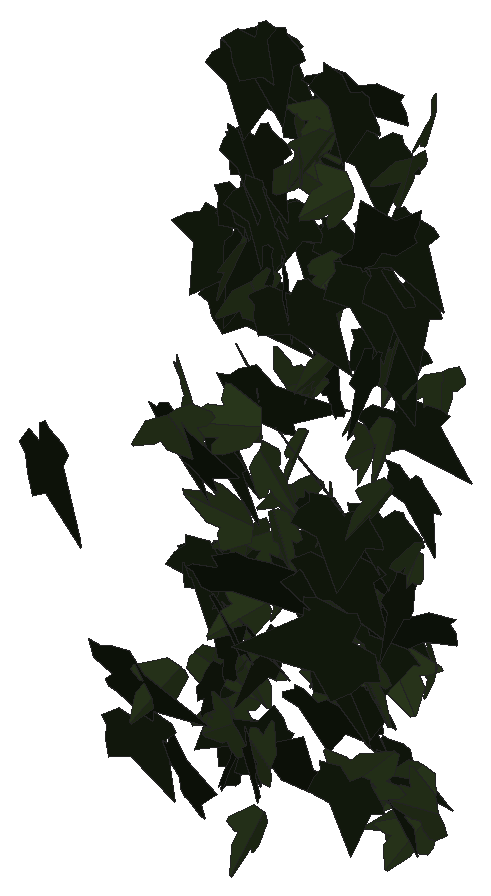
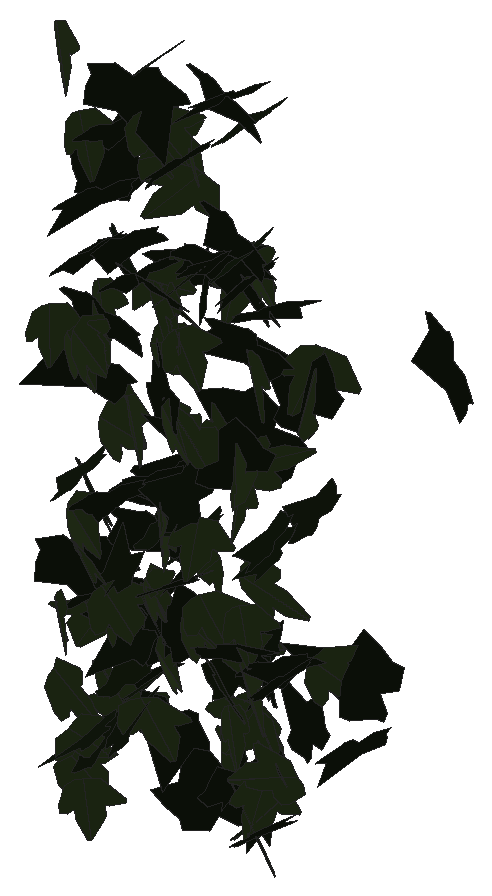
# SketchUp Ruby script. Lengths in inches.
U = 1.inch
M = Sketchup.active_model
def pt(a) = Geom::Point3d.new(a.map { |v| v * U })
def face(e, loops, mat)
  f = e.add_face(loops[0].map { |a| pt(a) })
  loops[1..].each { |l| e.add_face(l.map { |a| pt(a) }).erase! }
  f.material = f.back_material = mat if mat
  f
end
# faces: each face lists its corners as indices into pts; further lists are holes
def faces(e, pts, list, mat = nil) = list.each { |f| face(e, (f[0].is_a?(Array) ? f : [f]).map { |l| l.map { |i| pts[i] } }, mat) }
# xy, xz, yz: faces in a plane at the given z, y or x. An outline is a flat list of corners, or four numbers for a rectangle; further outlines are holes
def ring(l) = l.size == 4 ? [[l[0], l[1]], [l[2], l[1]], [l[2], l[3]], [l[0], l[3]]] : l.each_slice(2).to_a
def flat(e, list, mat, &to3) = list.each { |f| face(e, (f[0].is_a?(Array) ? f : [f]).map { |l| ring(l).map { |u, v| to3.(u, v) } }, mat) }
def xy(e, z, list, mat = nil) = flat(e, list, mat) { |x, y| [x, y, z] }
def xz(e, y, list, mat = nil) = flat(e, list, mat) { |x, z| [x, y, z] }
def yz(e, x, list, mat = nil) = flat(e, list, mat) { |y, z| [x, y, z] }
def lines(e, pts, list) = list.each { |a, b| e.add_line(pt(pts[a]), pt(pts[b])) }
# prism: a flat outline (further loops are holes) pulled along v
def prism(e, loops, v, mat = nil)
  f = face(e, loops, mat); d = Geom::Vector3d.new(v.map { |x| x * U })
  f.pushpull(f.normal.samedirection?(d) ? d.length : -d.length)
end
def box(e, o, s, mat = nil) = prism(e, [[o, [o[0] + s[0], o[1], o[2]], [o[0] + s[0], o[1] + s[1], o[2]], [o[0], o[1] + s[1], o[2]]]], [0, 0, s[2]], mat)
def at(x, y, z, deg = 0) = Geom::Transformation.translation(pt([x, y, z])) * Geom::Transformation.rotation(ORIGIN, Z_AXIS, deg.degrees)
def axes(o, x, y, z) = Geom::Transformation.new([*x, 0, *y, 0, *z, 0, *pt(o).to_a, 1])
def part(name) = M.definitions.add(name)
# library, detail: a bought-in or finely detailed component or shape, given as its bounding box
def library(name, o, s) = part(name).tap { |d| box(d.entities, o, s) }
def detail(e, o, s) = box(e.add_group.entities, o, s)
def put(e, d, t, mat = nil) = e.add_instance(d, t).tap { |i| i.material = mat if mat }
def group(e, t, mat = nil) = e.add_group.tap { |g| g.transformation = t; g.material = mat if mat }.entities
root = M.entities
M.materials.add("1026 AP 7946 SUNNY SIDE UP").color = [254, 231, 186]
M.materials.add("efeu1").color = [18, 25, 13]
M.materials.add("efeu2").color = [43, 57, 29]
c1 = part("ivyleaf_9")
p = [[1.54,2.16,1.25],[1.36,2.04,1.19],[-0.21,0.99,0.68],[-0.71,1.11,0.82],[-0.85,0.86,0.67],[-0.8,0.17,0.21],
  [-0.9,-0.01,0.1],[-0.67,-0.16,-0.02],[-0.08,-0.08,-0.05],[-0.03,-0.6,-0.4],[0.65,-0.88,-0.66],[0.83,-0.6,-0.49],
  [1.29,-0.42,-0.43],[1.8125,-0.07,-0.26],[1.21,0.44,0.15]]
faces(c1.entities,p,[[0,1,2,3,4,5,6,7,8,9,10,11,12,13,14]],"efeu1")
c2 = part("ivyleaf_10")
p = [[0,0.5,-0.03],[-0.0625,2.02,-0.43],[-0.19,2.01,-0.46],[-0.54,1.05,-0.29],[-0.52,0.625,-0.18],[-0.83,0.76,-0.28],
  [-1.16,0.64,-0.33],[-1.15,0.33,-0.24],[-0.77,-0.39,0.02],[-0.3,-0.51,0.16],[0.04,-0.48,0.23],[-0.02,2.01,-0.4375],
  [-0.06,2.01,-0.43],[0.04,-0.49,0.23],[0.67,-0.49,0.14],[1.38,0.36,-0.2],[1.375,0.51,-0.24],[0.81,0.65,-0.19],
  [0.62,0.59,-0.15],[0.6,1.09,-0.28],[0.5,1.23,-0.31]]
faces(c2.entities,p,[[0,1,2,3,4,5,6,7,8,9,10],[11,12,0,13,14,15,16,17,18,19,20]],"efeu2")
put(root,c1,axes([121.61,208.34,285.75],[-0.09102,-0.03713,-0.47993],[0.72895,-0.06226,-0.05462],[-0.09031,-0.46509,0.04284]),"1026 AP 7946 SUNNY SIDE UP")
put(root,c1,axes([124.05,209.3,284.24],[0.61403,0.15623,0.13736],[0.21568,0.01226,-0.43147],[-0.23915,0.41217,-0.03647]),"1026 AP 7946 SUNNY SIDE UP")
put(root,c2,axes([124.125,209.9,279.97],[-0.01613,-0.25056,0.28133],[0.13214,-0.26906,-0.25135],[0.56927,0.05536,0.06631]),"1026 AP 7946 SUNNY SIDE UP")
put(root,c1,axes([125.59,210.1,283.27],[-0.05091,-0.26888,-0.37248],[-0.09121,-0.35545,0.27677],[-0.70066,0.06581,-0.00896]),"1026 AP 7946 SUNNY SIDE UP")
put(root,c2,axes([122.8,209.76,285.93],[-0.33022,-0.28248,-0.17885],[0.18974,0.12426,-0.36128],[0.48418,-0.24135,0.0196]),"1026 AP 7946 SUNNY SIDE UP")
put(root,c1,axes([122.71,210.06,280.16],[0.05579,-0.04879,0.37356],[0.17873,-0.34511,-0.06127],[0.5473,0.11767,-0.01807]),"1026 AP 7946 SUNNY SIDE UP")
put(root,c1,axes([122.64,210.1,285.39],[0.10603,-0.13519,0.41887],[0.32724,-0.35034,-0.15732],[0.59024,0.21852,0.01198]),"1026 AP 7946 SUNNY SIDE UP")
put(root,c1,axes([121.55,210.08,281.34],[0.32519,-0.12393,0.35637],[0.40668,-0.234,-0.24653],[0.41189,0.32888,-0.03794]),"1026 AP 7946 SUNNY SIDE UP")
put(root,c2,axes([122.31,210.27,281.5],[-0.11299,-0.24724,0.28312],[0.00223,-0.28155,-0.26088],[0.58291,-0.04684,0.05588]),"1026 AP 7946 SUNNY SIDE UP")
put(root,c1,axes([121.69,210.31,280.56],[0.08574,-0.31958,-0.16892],[-0.03577,0.1606,-0.33303],[0.56236,0.05894,0.00457]),"1026 AP 7946 SUNNY SIDE UP")
put(root,c1,axes([125.13,210.74,280.59],[-0.08001,-0.32564,0.01922],[-0.0008,-0.02068,-0.33965],[0.51305,-0.05081,0.00247]),"1026 AP 7946 SUNNY SIDE UP")
put(root,c1,axes([125.38,210.9,287.25],[-0.30488,0.04205,-0.31612],[0.42375,-0.15608,-0.19822],[-0.24078,-0.32793,0.05142]),"1026 AP 7946 SUNNY SIDE UP")
put(root,c2,axes([122.25,210.77,285.64],[-0.31836,0.30173,0.0568],[0.06922,-0.03472,0.37372],[0.47682,0.2065,-0.01633]),"1026 AP 7946 SUNNY SIDE UP")
put(root,c1,axes([123.96,211,283.3125],[0.12499,-0.33358,0.08934],[0.02003,-0.08804,-0.3537],[0.54235,0.08013,-0.00753]),"1026 AP 7946 SUNNY SIDE UP")
put(root,c2,axes([123.43,210.98,284.96],[0.17881,-0.04143,0.34507],[0.48767,-0.12721,-0.12534],[0.21025,0.3303,-0.00274]),"1026 AP 7946 SUNNY SIDE UP")
put(root,c2,axes([123.31,210.86,287.73],[-0.17253,-0.34111,-0.16611],[0.11104,0.14434,-0.36766],[0.58147,-0.12878,0.02092]),"1026 AP 7946 SUNNY SIDE UP")
put(root,c2,axes([122.92,210.86,280.68],[-0.27788,0.1153,0.25612],[-0.38362,0.06688,-0.21077],[-0.19422,-0.29706,0.04987]),"1026 AP 7946 SUNNY SIDE UP")
put(root,c1,axes([123.12,211.16,279.85],[-0.11226,0.0883,0.32367],[-0.09416,-0.31921,0.07666],[0.50368,-0.03999,0.08647]),"1026 AP 7946 SUNNY SIDE UP")
put(root,c2,axes([122.85,211.11,288.04],[0.14731,-0.33648,0.0969],[0.03265,-0.09383,-0.36034],[0.54921,0.09583,-0.00457]),"1026 AP 7946 SUNNY SIDE UP")
put(root,c1,axes([124.27,211.32,282.44],[-0.11251,-0.16508,0.3382],[-0.17941,-0.30894,-0.18694],[0.55061,-0.1344,0.00819]),"1026 AP 7946 SUNNY SIDE UP")
put(root,c1,axes([122.62,211.26,281.99],[-0.00972,-0.15483,0.29514],[0.08362,-0.28406,-0.15815],[0.50641,0.04393,0.03178]),"1026 AP 7946 SUNNY SIDE UP")
put(root,c1,axes([123.89,211.04,287.7],[-0.08042,-0.21821,-0.29571],[0.23162,0.25063,-0.22283],[0.51579,-0.14657,0.05396]),"1026 AP 7946 SUNNY SIDE UP")
put(root,c1,axes([125.73,211.19,283.64],[-0.34251,0.07972,-0.26507],[0.36347,-0.11571,-0.23879],[-0.2188,-0.31702,0.01828]),"1026 AP 7946 SUNNY SIDE UP")
put(root,c1,axes([122.57,211.18,281.49],[-0.07866,0.1721,0.28129],[0.04264,-0.2721,0.18086],[0.5044,0.04984,0.02858]),"1026 AP 7946 SUNNY SIDE UP")
put(root,c2,axes([125.02,211.21,282.23],[-0.35779,0.22008,-0.21852],[0.20305,-0.17217,-0.32583],[-0.43712,-0.26011,0.02751]),"1026 AP 7946 SUNNY SIDE UP")
put(root,c1,axes([121.57,211.33,284.63],[0.18205,-0.29227,0.14544],[0.0786,-0.13383,-0.32463],[0.50543,0.12608,-0.00191]),"1026 AP 7946 SUNNY SIDE UP")
put(root,c1,axes([123.53,211.4,287.3],[-0.01971,0.02165,0.38698],[-0.06805,-0.37331,0.0185],[0.58752,-0.04251,0.01513]),"1026 AP 7946 SUNNY SIDE UP")
put(root,c2,axes([125.13,211.41,284.87],[0.04592,-0.23723,0.27759],[0.04198,-0.26951,-0.24778],[0.56453,0.03934,-0.00415]),"1026 AP 7946 SUNNY SIDE UP")
put(root,c2,axes([124.37,211.47,289.33],[-0.1084,-0.02226,0.36682],[0.06144,-0.36107,-0.01757],[0.5578,0.03544,0.07322]),"1026 AP 7946 SUNNY SIDE UP")
put(root,c2,axes([122.66,211.45,285.09],[-0.0318,0.11349,0.38625],[-0.16041,-0.36334,0.10569],[0.5937,-0.09209,0.04924]),"1026 AP 7946 SUNNY SIDE UP")
put(root,c2,axes([122.85,211.48,282.24],[-0.11298,-0.10099,0.33685],[-0.03896,-0.33227,-0.11308],[0.53756,-0.04531,0.0626]),"1026 AP 7946 SUNNY SIDE UP")
put(root,c1,axes([122.92,211.375,287.95],[-0.46652,0.03473,-0.23776],[0.35274,-0.0617,-0.30676],[-0.10236,-0.37091,0.02652]),"1026 AP 7946 SUNNY SIDE UP")
put(root,c1,axes([124.46,211.4375,284.27],[-0.19498,-0.32406,-0.01834],[0.0232,0.01144,-0.35725],[0.50965,-0.1245,0.00924]),"1026 AP 7946 SUNNY SIDE UP")
put(root,c2,axes([124.9,211.26,280.34],[-0.46007,-0.10063,0.17273],[0.23059,0.08822,0.31762],[-0.20455,0.32578,-0.03043]),"1026 AP 7946 SUNNY SIDE UP")
put(root,c2,axes([123.67,211.45,285.16],[0.26307,-0.30067,0.14705],[0.08531,-0.13491,-0.35484],[0.51752,0.17508,-0.01626]),"1026 AP 7946 SUNNY SIDE UP")
put(root,c2,axes([123.38,211.11,280.17],[0.07023,0.03151,0.37937],[-0.49688,0.19531,0.02342],[-0.30089,-0.31517,0.04988]),"1026 AP 7946 SUNNY SIDE UP")
put(root,c2,axes([124.07,211.59,286.59],[0.04814,-0.08331,0.37593],[0.13547,-0.35522,-0.09295],[0.57349,0.0909,-0.0096]),"1026 AP 7946 SUNNY SIDE UP")
put(root,c2,axes([125.22,211.42,285.89],[0.33467,-0.24235,0.11131],[0.10141,-0.08893,-0.33266],[0.40563,0.22219,-0.00867]),"1026 AP 7946 SUNNY SIDE UP")
put(root,c2,axes([126.18,211.2,280.34],[-0.19311,0.05531,0.37011],[-0.55424,0.07316,-0.13543],[-0.13763,-0.37225,0.02607]),"1026 AP 7946 SUNNY SIDE UP")
put(root,c1,axes([125.12,211.46,288.7],[0.25256,0.17382,0.33773],[-0.39064,-0.21352,0.24151],[0.43153,-0.29502,0.02096]),"1026 AP 7946 SUNNY SIDE UP")
put(root,c2,axes([124.34,211.43,282.6],[0.22254,-0.3072,0.06021],[0.01862,-0.06076,-0.34849],[0.49188,0.14129,-0.01405]),"1026 AP 7946 SUNNY SIDE UP")
put(root,c1,axes([122.79,211.54,281.7],[0.45271,-0.21313,-0.08655],[0.13142,-0.02584,0.36773],[-0.33465,-0.29847,0.02733]),"1026 AP 7946 SUNNY SIDE UP")
put(root,c1,axes([124.32,211.38,283.48],[-0.12408,-0.16562,-0.31602],[0.40093,0.18571,-0.1703],[0.3719,-0.25547,0.07816]),"1026 AP 7946 SUNNY SIDE UP")
put(root,c1,axes([122.6,211.67,290.54],[-0.07719,-0.32886,0.16903],[0.02267,-0.169,-0.34162],[0.57877,-0.03724,0.03593]),"1026 AP 7946 SUNNY SIDE UP")
put(root,c1,axes([124.39,211.66,290.82],[-0.05839,-0.33295,0.15199],[-0.01346,-0.14936,-0.34592],[0.57368,-0.03739,0.00735]),"1026 AP 7946 SUNNY SIDE UP")
put(root,c1,axes([122.24,211.72,287.8],[-0.30862,-0.27455,0.11321],[-0.03626,-0.11913,-0.34485],[0.46451,-0.19171,0.0483]),"1026 AP 7946 SUNNY SIDE UP")
put(root,c2,axes([123.875,211.66,289.89],[-0.01015,-0.2992,0.21085],[0.00111,-0.20641,-0.30949],[0.57152,-0.00492,0.00435]),"1026 AP 7946 SUNNY SIDE UP")
put(root,c1,axes([123.11,211.59,281.64],[-0.40042,0.10925,-0.19393],[0.25342,-0.10149,-0.28494],[-0.23127,-0.30037,0.02356]),"1026 AP 7946 SUNNY SIDE UP")
put(root,c2,axes([123.45,211.73,289.86],[0.10528,-0.13276,0.36696],[0.37768,-0.26654,-0.1501],[0.46473,0.24669,0.03885]),"1026 AP 7946 SUNNY SIDE UP")
put(root,c1,axes([121.99,211.51,280.55],[-0.08609,0.30228,0.20241],[0.00869,-0.19628,0.31429],[0.56536,0.04905,0.02599]),"1026 AP 7946 SUNNY SIDE UP")
put(root,c2,axes([124.83,211.45,285.49],[0.20352,-0.22938,-0.22112],[-0.17587,0.18177,-0.27019],[0.46008,0.17095,-0.00547]),"1026 AP 7946 SUNNY SIDE UP")
put(root,c1,axes([122.9,211.72,279.89],[0.00085,0.07128,0.35002],[-0.41781,-0.21796,0.04633],[0.35034,-0.26011,0.0544]),"1026 AP 7946 SUNNY SIDE UP")
put(root,c1,axes([124.76,211.67,288.01],[-0.11089,-0.34066,-0.08999],[0.02455,0.08399,-0.35789],[0.55169,-0.07221,-0.00216]),"1026 AP 7946 SUNNY SIDE UP")
put(root,c2,axes([125.51,211.71,279.55],[-0.22792,-0.20854,0.18715],[-0.04312,-0.19453,-0.25209],[0.43397,-0.12885,0.07324]),"1026 AP 7946 SUNNY SIDE UP")
put(root,c1,axes([122.49,211.58,287.11],[0.01902,-0.15223,-0.33054],[0.42386,0.21178,-0.09206],[0.36167,-0.24019,0.12527]),"1026 AP 7946 SUNNY SIDE UP")
put(root,c1,axes([122.55,211.35,279.84],[-0.07895,0.08404,-0.33801],[-0.38036,0.22396,0.0984],[0.37381,0.24563,0.02873]),"1026 AP 7946 SUNNY SIDE UP")
put(root,c1,axes([125.01,211.82,279.99],[0.13234,-0.29008,0.17996],[0.06814,-0.171,-0.31212],[0.52942,0.09452,-0.00481]),"1026 AP 7946 SUNNY SIDE UP")
put(root,c2,axes([123.11,211.73,283.57],[-0.30925,0.16677,-0.21142],[0.14687,-0.19667,-0.25683],[-0.39023,-0.20618,0.07088]),"1026 AP 7946 SUNNY SIDE UP")
put(root,c1,axes([123.85,211.88,283.79],[-0.04977,-0.2591,0.21968],[0.07517,-0.21694,-0.26369],[0.52375,0.00651,0.05872]),"1026 AP 7946 SUNNY SIDE UP")
put(root,c2,axes([125.13,211.61,287],[0.02635,-0.34587,-0.08812],[0.00833,0.0839,-0.35611],[0.55943,0.01504,0.00945]),"1026 AP 7946 SUNNY SIDE UP")
put(root,c2,axes([124.11,211.77,282.79],[0.08237,-0.29865,0.1291],[0.04861,-0.12348,-0.31297],[0.50798,0.06024,0.00901]),"1026 AP 7946 SUNNY SIDE UP")
put(root,c1,axes([122.83,211.81,291.02],[-0.27387,-0.11629,-0.31942],[0.51405,-0.00911,-0.18612],[0.07653,-0.35493,0.10713]),"1026 AP 7946 SUNNY SIDE UP")
put(root,c2,axes([124.18,211.78,282.5],[0.29717,-0.27858,0.10956],[0.07431,-0.09823,-0.34702],[0.46385,0.19421,-0.0146]),"1026 AP 7946 SUNNY SIDE UP")
put(root,c1,axes([125,211.9,282.47],[-0.19437,-0.33518,0.06312],[-0.0174,-0.06322,-0.36822],[0.53604,-0.12359,0.01094]),"1026 AP 7946 SUNNY SIDE UP")
put(root,c2,axes([122.54,211.66,281.28],[-0.51237,0.03659,-0.09911],[0.14306,-0.0484,-0.33599],[-0.07633,-0.33635,0.03553]),"1026 AP 7946 SUNNY SIDE UP")
put(root,c1,axes([123.01,211.75,279.66],[0.58099,0.01898,0.04167],[-0.06602,0.03497,0.37946],[0.02357,-0.37004,0.03581]),"1026 AP 7946 SUNNY SIDE UP")
put(root,c1,axes([123.39,211.76,282.4],[0.3876,-0.17388,0.18358],[0.19929,-0.1298,-0.31015],[0.33826,0.27572,-0.02762]),"1026 AP 7946 SUNNY SIDE UP")
put(root,c1,axes([122.99,211.83,288.46],[-0.40203,-0.21455,-0.13333],[0.17867,0.06358,-0.34268],[0.35004,-0.27887,0.02177]),"1026 AP 7946 SUNNY SIDE UP")
put(root,c1,axes([122.92,211.92,288.45],[-0.17334,-0.35542,0.05624],[-0.00708,-0.05784,-0.38347],[0.56586,-0.1096,0.01243]),"1026 AP 7946 SUNNY SIDE UP")
put(root,c1,axes([124.45,211.95,281.29],[-0.05274,-0.25382,0.22511],[0.09156,-0.2221,-0.25618],[0.52012,0.01336,0.06793]),"1026 AP 7946 SUNNY SIDE UP")
put(root,c2,axes([123.98,211.91,287.77],[0.18652,0.18334,-0.31227],[-0.20083,-0.27719,-0.22507],[-0.52106,0.17247,-0.02503]),"1026 AP 7946 SUNNY SIDE UP")
put(root,c1,axes([125.41,211.6875,282.88],[0.19132,0.25939,-0.25064],[-0.16249,-0.22188,-0.29646],[-0.53673,0.15963,0.00041]),"1026 AP 7946 SUNNY SIDE UP")
put(root,c1,axes([122.73,211.73,291.0625],[0.16667,-0.31036,-0.17256],[0.0641,0.18277,-0.32464],[0.54951,0.07282,0.09021]),"1026 AP 7946 SUNNY SIDE UP")
put(root,c1,axes([121.96,211.85,284.33],[0.24895,-0.30809,0.04118],[-0.00109,-0.04717,-0.3564],[0.48886,0.15679,-0.02177]),"1026 AP 7946 SUNNY SIDE UP")
put(root,c2,axes([122.41,211.64,283.43],[0.05269,-0.05233,-0.37419],[-0.49069,0.18729,-0.05641],[0.30274,0.31267,-0.0263]),"1026 AP 7946 SUNNY SIDE UP")
put(root,c2,axes([123.99,211.92,290.23],[-0.31514,-0.24954,0.21582],[-0.05894,-0.22823,-0.31622],[0.51036,-0.18045,0.09674]),"1026 AP 7946 SUNNY SIDE UP")
put(root,c1,axes([124.79,211.89,284.11],[-0.08422,-0.33481,-0.07406],[0.01673,0.06917,-0.3489],[0.53757,-0.05461,-0.00075]),"1026 AP 7946 SUNNY SIDE UP")
put(root,c1,axes([121.86,211.93,282.47],[-0.21033,-0.30231,-0.02575],[0.02624,0.01807,-0.34036],[0.47604,-0.13457,0.00738]),"1026 AP 7946 SUNNY SIDE UP")
put(root,c2,axes([125.05,211.74,282.07],[0.41265,0.20671,0.11985],[0.16837,0.04961,-0.34283],[-0.33179,0.28226,-0.02492]),"1026 AP 7946 SUNNY SIDE UP")
put(root,c2,axes([123.79,211.93,281.88],[0.21534,-0.25891,0.15959],[0.09592,-0.14449,-0.30233],[0.46583,0.14944,-0.01152]),"1026 AP 7946 SUNNY SIDE UP")
put(root,c1,axes([123.96,211.88,281.5],[0.14282,-0.32877,-0.03614],[0.0013,0.03467,-0.35103],[0.51958,0.09028,0.01081]),"1026 AP 7946 SUNNY SIDE UP")
put(root,c2,axes([123.52,211.68,289.35],[-0.29828,-0.18329,-0.25273],[0.31344,0.14355,-0.2696],[0.36381,-0.27396,0.02506]),"1026 AP 7946 SUNNY SIDE UP")
put(root,c1,axes([122.1,211.83,279.35],[-0.05393,0.23758,0.25356],[0.06013,-0.24178,0.24586],[0.53299,0.05132,-0.00208]),"1026 AP 7946 SUNNY SIDE UP")
put(root,c1,axes([125.16,211.75,285.99],[-0.05597,-0.10452,-0.35024],[0.34978,0.2593,-0.10479],[0.43524,-0.22183,0.03917]),"1026 AP 7946 SUNNY SIDE UP")
put(root,c1,axes([123.21,211.97,284.6],[0.32359,-0.27741,0.18813],[0.15198,-0.15744,-0.35646],[0.50106,0.22691,-0.01338]),"1026 AP 7946 SUNNY SIDE UP")
put(root,c2,axes([125.75,211.75,290.91],[0.10846,-0.33081,-0.15435],[-0.03012,0.14707,-0.34711],[0.56902,0.07084,0.01105]),"1026 AP 7946 SUNNY SIDE UP")
put(root,c1,axes([125.07,211.98,287.86],[-0.00018,-0.37814,-0.00665],[-0.00923,0.00431,-0.38949],[0.59456,-0.00005,-0.00605]),"1026 AP 7946 SUNNY SIDE UP")
put(root,c1,axes([122.3125,211.9,288.36],[0.12922,-0.33587,-0.08022],[-0.0534,0.06981,-0.35543],[0.53882,0.08747,-0.01599]),"1026 AP 7946 SUNNY SIDE UP")
put(root,c1,axes([124.86,211.92,286.94],[-0.26399,-0.11801,-0.3021],[0.45557,0.07349,-0.20138],[0.19631,-0.32923,0.06107]),"1026 AP 7946 SUNNY SIDE UP")
put(root,c1,axes([122.54,211.81,285.26],[0.14249,-0.01639,0.37272],[0.53602,-0.12239,-0.09436],[0.19277,0.35242,-0.01312]),"1026 AP 7946 SUNNY SIDE UP")
put(root,c1,axes([124.64,211.99,290.01],[-0.12386,-0.35145,-0.0313],[0.01604,0.0268,-0.37086],[0.55419,-0.07932,0.00374]),"1026 AP 7946 SUNNY SIDE UP")
put(root,c1,axes([123.69,212.09,283.11],[-0.25159,-0.24643,0.15311],[-0.03488,-0.16054,-0.29697],[0.4523,-0.14945,0.06227]),"1026 AP 7946 SUNNY SIDE UP")
put(root,c2,axes([124.62,211.96,282.33],[0.02339,-0.30659,0.13517],[0.04883,-0.13123,-0.31613],[0.52318,0.02596,0.02346]),"1026 AP 7946 SUNNY SIDE UP")
put(root,c2,axes([123.21,212.04,282.64],[0.05084,-0.26379,0.22692],[0.044,-0.22,-0.27507],[0.5401,0.04275,0.00105]),"1026 AP 7946 SUNNY SIDE UP")
put(root,c1,axes([123.79,211.95,285.77],[-0.2023,0.16031,0.29591],[0.02922,-0.3035,0.18188],[0.51516,0.08017,0.10589]),"1026 AP 7946 SUNNY SIDE UP")
put(root,c1,axes([123.76,211.78,280.91],[0.44051,0.071,-0.19825],[-0.28415,-0.07013,-0.29746],[-0.15386,0.3328,-0.01826]),"1026 AP 7946 SUNNY SIDE UP")
put(root,c2,axes([123.875,211.72,287.41],[0.20212,-0.194,-0.28133],[-0.15224,0.25728,-0.23469],[0.50276,0.1559,0.04203]),"1026 AP 7946 SUNNY SIDE UP")
put(root,c2,axes([125.27,212.01,280.22],[0.14834,0.20907,-0.23113],[-0.232,-0.17622,-0.23289],[-0.42428,0.16946,0.04654]),"1026 AP 7946 SUNNY SIDE UP")
put(root,c2,axes([125.22,212.05,283.68],[0.09943,-0.33712,0.16518],[0.06337,-0.15746,-0.35414],[0.58487,0.07437,0.01029]),"1026 AP 7946 SUNNY SIDE UP")
put(root,c2,axes([122.13,211.83,280.31],[-0.26472,-0.27625,-0.12242],[0.12554,0.08838,-0.33207],[0.45489,-0.18516,0.0204]),"1026 AP 7946 SUNNY SIDE UP")
put(root,c1,axes([121.99,211.98,280.08],[0.16713,-0.3034,-0.04542],[-0.03169,0.03782,-0.3309],[0.48065,0.10799,-0.00603]),"1026 AP 7946 SUNNY SIDE UP")
put(root,c1,axes([124.95,211.9,288.81],[0.10169,-0.33024,-0.20874],[-0.00125,0.20342,-0.34382],[0.60768,0.05568,0.03422]),"1026 AP 7946 SUNNY SIDE UP")
put(root,c1,axes([124.09,211.61,282.28],[-0.00266,0.28517,-0.25195],[-0.04649,0.24533,0.2944],[0.59055,0.0206,0.02204]),"1026 AP 7946 SUNNY SIDE UP")
put(root,c2,axes([122.3,211.83,286.98],[0.30142,-0.24996,-0.16642],[-0.07122,0.16375,-0.31823],[0.4613,0.18861,0.05961]),"1026 AP 7946 SUNNY SIDE UP")
put(root,c2,axes([123.23,211.89,284.07],[-0.2354,-0.28451,-0.10861],[0.08343,0.08937,-0.33063],[0.46884,-0.15875,0.0043]),"1026 AP 7946 SUNNY SIDE UP")
put(root,c1,axes([124.32,211.93,290.79],[0.3014,0.17823,-0.2774],[-0.27951,-0.20458,-0.27005],[-0.42548,0.26065,-0.0191]),"1026 AP 7946 SUNNY SIDE UP")
put(root,c1,axes([123.27,212.19,288.07],[-0.00478,-0.32923,0.1257],[-0.01133,-0.1238,-0.33985],[0.553,-0.00538,-0.00588]),"1026 AP 7946 SUNNY SIDE UP")
put(root,c1,axes([121.62,212.03,282.39],[0.1295,-0.34053,-0.10431],[-0.03135,0.09735,-0.36034],[0.55688,0.08467,0.00397]),"1026 AP 7946 SUNNY SIDE UP")
put(root,c2,axes([122.6,211.93,281.34],[0.00889,-0.3107,-0.09309],[-0.00947,0.08849,-0.31959],[0.50794,0.00709,-0.00433]),"1026 AP 7946 SUNNY SIDE UP")
put(root,c2,axes([125.15,212,289.82],[-0.10824,-0.35875,-0.01369],[0.01291,0.00988,-0.37621],[0.56423,-0.06905,0.00598]),"1026 AP 7946 SUNNY SIDE UP")
put(root,c1,axes([122.6,212.1875,282.55],[-0.42824,-0.16648,0.07349],[-0.05527,-0.07949,-0.32552],[0.27997,-0.27033,0.04814]),"1026 AP 7946 SUNNY SIDE UP")
put(root,c2,axes([122.92,212.09,283.05],[-0.23616,-0.26762,0.12016],[-0.05222,-0.11636,-0.31569],[0.45702,-0.15159,0.02602]),"1026 AP 7946 SUNNY SIDE UP")
put(root,c2,axes([122.4375,211.89,285],[0.07931,-0.30283,-0.19052],[0.0707,0.18905,-0.30805],[0.55202,0.01929,0.06682]),"1026 AP 7946 SUNNY SIDE UP")
put(root,c2,axes([121.67,211.94,280.76],[0.22832,-0.01537,0.29402],[0.421,0.11962,-0.13295],[-0.15768,0.29712,0.07076]),"1026 AP 7946 SUNNY SIDE UP")
put(root,c2,axes([125.71,212.02,286.61],[-0.18341,-0.3213,-0.02012],[0.08061,0.00003,-0.34863],[0.49952,-0.11798,0.04887]),"1026 AP 7946 SUNNY SIDE UP")
put(root,c2,axes([123.96,211.93,287.57],[0.32046,-0.26023,-0.18427],[-0.11778,0.16518,-0.33732],[0.481,0.21382,0.04016]),"1026 AP 7946 SUNNY SIDE UP")
put(root,c2,axes([122.33,212.02,283.05],[-0.14617,-0.3132,-0.01606],[0.01002,0.01251,-0.33648],[0.49285,-0.09314,0.00208]),"1026 AP 7946 SUNNY SIDE UP")
put(root,c2,axes([123.9,211.83,283.96],[0.04772,-0.19674,-0.29839],[-0.10954,0.28038,-0.20286],[0.53808,0.07453,-0.01483]),"1026 AP 7946 SUNNY SIDE UP")
put(root,c1,axes([124.41,212.26,283],[-0.14037,-0.10062,0.31391],[0.04795,-0.31805,-0.10067],[0.50314,0.00224,0.09717]),"1026 AP 7946 SUNNY SIDE UP")
put(root,c2,axes([124.91,212.21,286.61],[-0.0242,-0.26433,0.2239],[0.10089,-0.21741,-0.26716],[0.53007,0.02931,0.06107]),"1026 AP 7946 SUNNY SIDE UP")
put(root,c2,axes([123.35,212.1,287.07],[-0.15389,-0.31536,0.07834],[-0.01663,-0.07815,-0.34037],[0.51048,-0.09762,0.01253]),"1026 AP 7946 SUNNY SIDE UP")
put(root,c1,axes([122.2,212.26,288.86],[0.01698,-0.32741,0.14232],[0.00089,-0.14005,-0.33827],[0.55991,0.01015,-0.00378]),"1026 AP 7946 SUNNY SIDE UP")
put(root,c1,axes([121.96,212.29,279.88],[-0.23362,-0.19647,0.21183],[-0.10875,-0.20133,-0.24949],[0.43507,-0.15582,0.05139]),"1026 AP 7946 SUNNY SIDE UP")
put(root,c1,axes([122.34,212.16,289.16],[-0.18758,-0.08454,-0.34662],[0.53796,0.02726,-0.13205],[0.08586,-0.35549,0.0701]),"1026 AP 7946 SUNNY SIDE UP")
put(root,c1,axes([124.88,211.96,280.41],[0.35196,-0.17724,-0.15688],[-0.08264,0.16596,-0.27945],[0.35696,0.21318,0.08999]),"1026 AP 7946 SUNNY SIDE UP")
put(root,c1,axes([123.32,212.14,290.01],[0.10431,-0.34409,-0.08518],[-0.00348,0.08173,-0.36028],[0.55573,0.06509,0.01373]),"1026 AP 7946 SUNNY SIDE UP")
put(root,c2,axes([123.96,212.11,281.06],[-0.42965,-0.0811,0.16051],[-0.21874,-0.07738,-0.29242],[0.16969,-0.30511,0.02947]),"1026 AP 7946 SUNNY SIDE UP")
put(root,c1,axes([124,212.2,287.89],[-0.52609,0.01424,-0.0738],[0.10746,-0.05854,-0.34076],[-0.04088,-0.33713,0.05402]),"1026 AP 7946 SUNNY SIDE UP")
put(root,c2,axes([123.49,212.17,285.86],[0.11405,-0.32064,0.06523],[0.01378,-0.0648,-0.339],[0.51429,0.07284,-0.00538]),"1026 AP 7946 SUNNY SIDE UP")
put(root,c2,axes([122.17,212.11,282.2],[0.1833,-0.34661,-0.04437],[-0.0253,0.03795,-0.37649],[0.54824,0.11764,-0.00254]),"1026 AP 7946 SUNNY SIDE UP")
put(root,c2,axes([125.03,212.11,279.42],[-0.24532,-0.27925,0.00291],[0.01374,-0.00993,-0.32934],[0.43894,-0.15576,0.01193]),"1026 AP 7946 SUNNY SIDE UP")
put(root,c1,axes([121.61,212.15,284.45],[0.29453,-0.28191,-0.04829],[-0.04992,0.03325,-0.34839],[0.44617,0.18982,-0.0071]),"1026 AP 7946 SUNNY SIDE UP")
put(root,c2,axes([122.98,212.16,285.52],[-0.33743,0.08166,0.27198],[0.41566,-0.03478,0.23264],[0.12426,0.33808,-0.03964]),"1026 AP 7946 SUNNY SIDE UP")
put(root,c2,axes([124.21,212.1,285.7],[0.13173,-0.32784,-0.10312],[-0.01888,0.09826,-0.34779],[0.53781,0.08375,0.01305]),"1026 AP 7946 SUNNY SIDE UP")
put(root,c2,axes([125.11,212.23,286.48],[0.05517,-0.33062,0.07394],[0.00006,-0.07404,-0.34286],[0.53262,0.03425,-0.00762]),"1026 AP 7946 SUNNY SIDE UP")
put(root,c1,axes([124.4,212.24,280.5],[0.0648,-0.31786,0.11403],[0.01121,0.11413,0.33019],[-0.53007,-0.03644,0.02092]),"1026 AP 7946 SUNNY SIDE UP")
put(root,c1,axes([124.11,212.07,282.27],[0.47525,-0.08523,-0.09443],[-0.124,0.05476,-0.32171],[0.15213,0.31092,0.03279]),"1026 AP 7946 SUNNY SIDE UP")
put(root,c2,axes([124.88,212.36,286.6875],[0.06711,-0.32171,0.2233],[0.10282,-0.21083,-0.33405],[0.60286,0.07177,0.03212]),"1026 AP 7946 SUNNY SIDE UP")
put(root,c2,axes([122.17,212.33,285.2],[-0.28543,0.12383,0.28149],[0.29488,-0.20139,0.22177],[0.36689,0.2582,0.04075]),"1026 AP 7946 SUNNY SIDE UP")
put(root,c2,axes([124.96,212.3,283.35],[0.38895,-0.20434,0.12408],[0.10665,-0.10755,-0.32894],[0.35837,0.25378,-0.03677]),"1026 AP 7946 SUNNY SIDE UP")
put(root,c2,axes([124.42,212.31,282.75],[-0.19311,-0.3223,0.16012],[-0.04747,-0.15634,-0.3553],[0.56189,-0.12397,0.02501]),"1026 AP 7946 SUNNY SIDE UP")
put(root,c1,axes([123.9375,212.34,288.08],[-0.05643,-0.34858,-0.01166],[0.01267,0.00855,-0.36088],[0.54816,-0.03608,0.00714]),"1026 AP 7946 SUNNY SIDE UP")
put(root,c2,axes([125.5625,212,282.07],[0.08936,-0.13778,-0.31186],[-0.14982,0.28666,-0.15155],[0.49989,0.11054,0.01033]),"1026 AP 7946 SUNNY SIDE UP")
put(root,c1,axes([124.91,212.36,284.55],[0.11919,-0.31893,0.08776],[0.02886,-0.08506,-0.33821],[0.51901,0.07797,-0.00135]),"1026 AP 7946 SUNNY SIDE UP")
